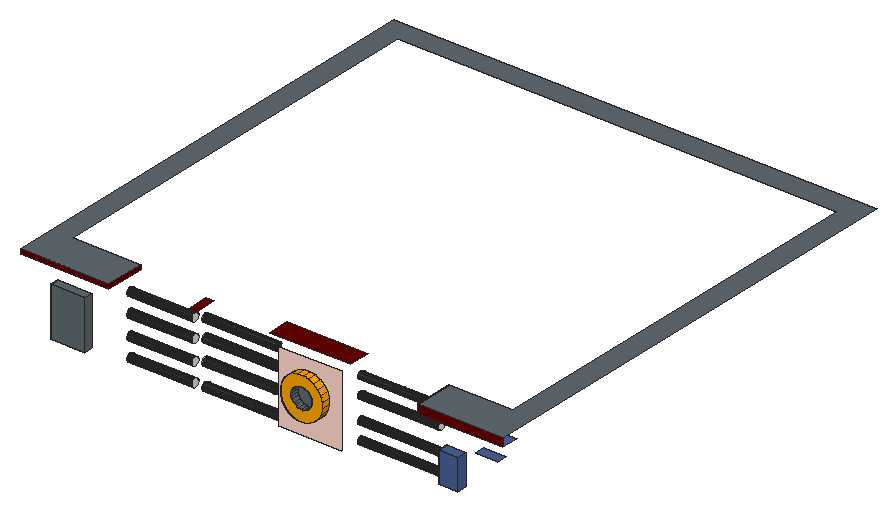
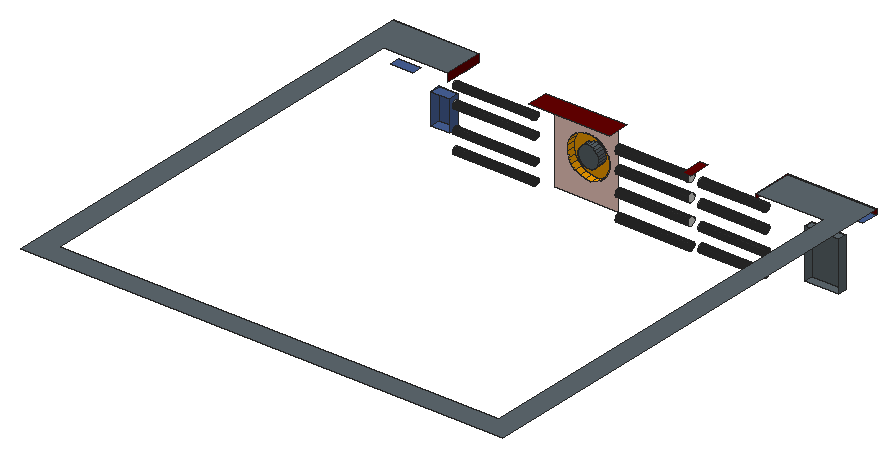
# SketchUp Ruby script. Lengths in inches.
U = 1.inch
M = Sketchup.active_model
def pt(a) = Geom::Point3d.new(a.map { |v| v * U })
def face(e, loops, mat)
  f = e.add_face(loops[0].map { |a| pt(a) })
  loops[1..].each { |l| e.add_face(l.map { |a| pt(a) }).erase! }
  f.material = f.back_material = mat if mat
  f
end
# faces: each face lists its corners as indices into pts; further lists are holes
def faces(e, pts, list, mat = nil) = list.each { |f| face(e, (f[0].is_a?(Array) ? f : [f]).map { |l| l.map { |i| pts[i] } }, mat) }
# xy, xz, yz: faces in a plane at the given z, y or x. An outline is a flat list of corners, or four numbers for a rectangle; further outlines are holes
def ring(l) = l.size == 4 ? [[l[0], l[1]], [l[2], l[1]], [l[2], l[3]], [l[0], l[3]]] : l.each_slice(2).to_a
def flat(e, list, mat, &to3) = list.each { |f| face(e, (f[0].is_a?(Array) ? f : [f]).map { |l| ring(l).map { |u, v| to3.(u, v) } }, mat) }
def xy(e, z, list, mat = nil) = flat(e, list, mat) { |x, y| [x, y, z] }
def xz(e, y, list, mat = nil) = flat(e, list, mat) { |x, z| [x, y, z] }
def yz(e, x, list, mat = nil) = flat(e, list, mat) { |y, z| [x, y, z] }
def lines(e, pts, list) = list.each { |a, b| e.add_line(pt(pts[a]), pt(pts[b])) }
# prism: a flat outline (further loops are holes) pulled along v
def prism(e, loops, v, mat = nil)
  f = face(e, loops, mat); d = Geom::Vector3d.new(v.map { |x| x * U })
  f.pushpull(f.normal.samedirection?(d) ? d.length : -d.length)
end
def box(e, o, s, mat = nil) = prism(e, [[o, [o[0] + s[0], o[1], o[2]], [o[0] + s[0], o[1] + s[1], o[2]], [o[0], o[1] + s[1], o[2]]]], [0, 0, s[2]], mat)
def at(x, y, z, deg = 0) = Geom::Transformation.translation(pt([x, y, z])) * Geom::Transformation.rotation(ORIGIN, Z_AXIS, deg.degrees)
def axes(o, x, y, z) = Geom::Transformation.new([*x, 0, *y, 0, *z, 0, *pt(o).to_a, 1])
def part(name) = M.definitions.add(name)
# library, detail: a bought-in or finely detailed component or shape, given as its bounding box
def library(name, o, s) = part(name).tap { |d| box(d.entities, o, s) }
def detail(e, o, s) = box(e.add_group.entities, o, s)
def put(e, d, t, mat = nil) = e.add_instance(d, t).tap { |i| i.material = mat if mat }
def group(e, t, mat = nil) = e.add_group.tap { |g| g.transformation = t; g.material = mat if mat }.entities
root = M.entities
M.materials.add("[0038_Orange]").color = [255, 165, 0]
M.materials.add("[Color A08]").color = [102, 0, 0]
M.materials.add("[Color B01]").color = [255, 216, 204]
M.materials.add("[Color M07]").color = [58, 58, 58]
M.materials.add("[Formica Blue]").color = [71, 97, 152]
M.materials.add("[Formica Speckled Grey]").color = [94, 105, 111]
xy(root,173.26,[[56.92,25.54,71.36,29.17]],"[Formica Speckled Grey]")
xy(root,176.39,[[221.42,24.73,229.42,29.17]],"[Formica Blue]")
xy(root,189.34,[[221.42,24.73,229.42,29.17]],"[Formica Blue]")
xy(root,193.75,[[236.96,24.73,246.46,29.17]],"[Formica Blue]")
xy(root,193.95,[[56.92,25.54,71.36,29.17]],"[Formica Speckled Grey]")
xy(root,200.34,[[198.48,33.52,198.76,33.56,199.01,33.66,199.23,33.83,199.4,34.05,199.51,34.31,199.55,34.58,199.51,34.86,199.4,35.12,199.23,35.34,199.01,35.5,198.76,35.61,198.48,35.65,198.21,35.61,197.95,35.5,197.73,35.34,197.5625,35.12,197.46,34.86,197.42,34.58,197.46,34.31,197.5625,34.05,197.73,33.83,197.95,33.66,198.21,33.56]])
xy(root,202.04,[[214.88,21.86,251.02,29.17]],"[Formica Blue]")
xy(root,202.625,[[112.25,29.17,115.75,38.27]],"[Color A08]")
xy(root,203.49,[[47,21.86,84.58,29.17]],"[Formica Blue]")
xy(root,205.625,[[146.64,29.17,180.76,38.27]],"[Color A08]")
xy(root,205.625,[[47,21.86,84.58,21.86,84.58,38.27,56.16,38.27,56.16,209.77,241.86,209.77,241.86,38.27,214.88,38.27,214.88,21.86,251.02,21.86,251.02,218.93,47,218.93]],"[Formica Speckled Grey]")
xz(root,21.86,[[214.88,202.04,251.02,205.625],[47,203.49,84.58,205.625]],"[Color A08]")
xz(root,24.73,[[221.42,176.39,229.42,189.34]],"[Formica Blue]")
xz(root,25.54,[[56.92,173.26,71.36,193.95]],"[Formica Speckled Grey]")
xz(root,25.67,[[[161.83,179.01,164.18,179.07,166.43,179.74,168.43,180.97,170.05,182.68,171.17,184.75,171.71,187.03,171.65,189.38,170.98,191.63,169.74,193.63,168.04,195.25,165.97,196.37,163.6875,196.91,161.34,196.85,159.09,196.17,157.08,194.94,155.47,193.24,154.35,191.17,153.81,188.89,153.87,186.54,154.54,184.29,155.77,182.28,157.48,180.67,159.55,179.55],[162.3,183.54,161.17,183.8,160.15,184.36,159.31,185.15,158.7,186.14,158.37,187.26,158.34,188.42,158.61,189.55,159.16,190.57,159.96,191.41,160.94,192.02,162.06,192.35,163.22,192.38,164.35,192.11,165.37,191.5625,166.21,190.76,166.82,189.77,167.15,188.66,167.18,187.5,166.91,186.37,166.36,185.35,165.5625,184.51,164.57,183.9,163.46,183.57]]],"[0038_Orange]")
xz(root,29.17,[[[150.55,171.54,176.84,201.71],[161.83,179.01,159.55,179.55,157.48,180.67,155.77,182.28,154.54,184.29,153.87,186.54,153.81,188.89,154.35,191.17,155.47,193.24,157.08,194.94,159.09,196.17,161.34,196.85,163.6875,196.91,165.97,196.37,168.04,195.25,169.74,193.63,170.98,191.63,171.65,189.38,171.71,187.03,171.17,184.75,170.05,182.68,168.43,180.97,166.43,179.74,164.18,179.07]]],"[Color B01]")
xz(root,29.17,[[162.3,183.54,163.46,183.57,164.57,183.9,165.5625,184.51,166.36,185.35,166.91,186.37,167.18,187.5,167.15,188.66,166.82,189.77,166.21,190.76,165.37,191.5625,164.35,192.11,163.22,192.38,162.06,192.35,160.94,192.02,159.96,191.41,159.16,190.57,158.61,189.55,158.34,188.42,158.37,187.26,158.7,186.14,159.31,185.15,160.15,184.36,161.17,183.8]],"[Formica Speckled Grey]")
yz(root,56.92,[[25.54,173.26,29.17,193.95]],"[Formica Speckled Grey]")
yz(root,71.36,[[25.54,173.26,29.17,193.95]],"[Formica Speckled Grey]")
yz(root,84.58,[[21.86,203.49,38.27,205.625]],"[Color A08]")
yz(root,112.25,[[32.81,171.26,33.23,171.3125,33.62,171.47,33.96,171.73,34.22,172.07,34.38,172.46,34.43,172.88,34.38,173.3,34.22,173.69,33.96,174.03,33.62,174.29,33.23,174.45,32.81,174.51,32.39,174.45,32,174.29,31.66,174.03,31.4,173.69,31.24,173.3,31.18,172.88,31.24,172.46,31.4,172.07,31.66,171.73,32,171.47,32.39,171.3125],[32.81,179.38,33.23,179.4375,33.62,179.6,33.96,179.86,34.22,180.19,34.38,180.59,34.43,181.01,34.38,181.43,34.22,181.82,33.96,182.16,33.62,182.41,33.23,182.58,32.81,182.63,32.39,182.58,32,182.41,31.66,182.16,31.4,181.82,31.24,181.43,31.18,181.01,31.24,180.59,31.4,180.19,31.66,179.86,32,179.6,32.39,179.4375],[32.81,188.01,33.23,188.0625,33.62,188.22,33.96,188.48,34.22,188.82,34.38,189.21,34.43,189.63,34.38,190.05,34.22,190.44,33.96,190.78,33.62,191.04,33.23,191.2,32.81,191.26,32.39,191.2,32,191.04,31.66,190.78,31.4,190.44,31.24,190.05,31.18,189.63,31.24,189.21,31.4,188.82,31.66,188.48,32,188.22,32.39,188.0625],[32.81,196.19,33.23,196.25,33.62,196.41,33.96,196.67,34.22,197.01,34.38,197.4,34.43,197.82,34.38,198.24,34.22,198.63,33.96,198.97,33.62,199.23,33.23,199.39,32.81,199.44,32.39,199.39,32,199.23,31.66,198.97,31.4,198.63,31.24,198.24,31.18,197.82,31.24,197.4,31.4,197.01,31.66,196.67,32,196.41,32.39,196.25]])
yz(root,115.75,[[33.57,180.44,33.15,180.5,32.76,180.66,32.42,180.92,32.17,181.26,32,181.65,31.95,182.07,32,182.49,32.17,182.88,32.42,183.22,32.76,183.48,33.15,183.64,33.57,183.69,33.99,183.64,34.39,183.48,34.72,183.22,34.98,182.88,35.14,182.49,35.2,182.07,35.14,181.65,34.98,181.26,34.72,180.92,34.39,180.66,33.99,180.5],[33.57,189.26,33.15,189.3125,32.76,189.47,32.42,189.73,32.17,190.07,32,190.46,31.95,190.88,32,191.3,32.17,191.69,32.42,192.03,32.76,192.29,33.15,192.45,33.57,192.51,33.99,192.45,34.39,192.29,34.72,192.03,34.98,191.69,35.14,191.3,35.2,190.88,35.14,190.46,34.98,190.07,34.72,189.73,34.39,189.47,33.99,189.3125],[33.57,196.94,33.15,197,32.76,197.16,32.42,197.42,32.17,197.76,32,198.15,31.95,198.57,32,198.99,32.17,199.38,32.42,199.72,32.76,199.98,33.15,200.14,33.57,200.19,33.99,200.14,34.39,199.98,34.72,199.72,34.98,199.38,35.14,198.99,35.2,198.57,35.14,198.15,34.98,197.76,34.72,197.42,34.39,197.16,33.99,197]])
yz(root,214.88,[[34.44,173.05,34.81,173.11,35.15,173.27,35.4375,173.51,35.66,173.82,35.79,174.17,35.82,174.54,35.76,174.91,35.6,175.25,35.36,175.54,35.05,175.76,34.7,175.89,34.33,175.92,33.96,175.86,33.62,175.7,33.33,175.46,33.11,175.16,32.98,174.8,32.95,174.43,33.01,174.06,33.17,173.72,33.41,173.43,33.71,173.21,34.07,173.08],[34.44,180.68,34.81,180.74,35.15,180.9,35.4375,181.14,35.66,181.44,35.79,181.8,35.82,182.17,35.76,182.54,35.6,182.88,35.36,183.17,35.05,183.38,34.7,183.51,34.33,183.55,33.96,183.48,33.62,183.33,33.33,183.09,33.11,182.78,32.98,182.43,32.95,182.06,33.01,181.69,33.17,181.34,33.41,181.06,33.71,180.84,34.07,180.71],[34.44,190.43,34.81,190.49,35.15,190.65,35.4375,190.89,35.66,191.19,35.79,191.55,35.82,191.92,35.76,192.29,35.6,192.63,35.36,192.92,35.05,193.13,34.7,193.26,34.33,193.3,33.96,193.23,33.62,193.08,33.33,192.84,33.11,192.53,32.98,192.18,32.95,191.81,33.01,191.44,33.17,191.09,33.41,190.81,33.71,190.59,34.07,190.46],[34.44,197.93,34.81,197.99,35.15,198.15,35.4375,198.39,35.66,198.69,35.79,199.05,35.82,199.42,35.76,199.79,35.6,200.13,35.36,200.42,35.05,200.63,34.7,200.76,34.33,200.8,33.96,200.73,33.62,200.58,33.33,200.34,33.11,200.03,32.98,199.68,32.95,199.31,33.01,198.94,33.17,198.59,33.41,198.31,33.71,198.09,34.07,197.96]])
yz(root,214.88,[[21.86,202.04,38.27,205.625]],"[Color A08]")
yz(root,221.42,[[24.73,176.39,29.17,189.34]],"[Formica Blue]")
yz(root,229.42,[[24.73,176.39,29.17,189.34]],"[Formica Blue]")
p = [[115.75,33.15,171],[115.75,33.57,170.94],[146.64,33.57,170.94],[146.64,33.15,171],[115.75,33.99,171],[146.64,33.99,171],
  [115.75,32.76,171.16],[146.64,32.76,171.16],[115.75,34.39,171.16],[146.64,34.39,171.16],[115.75,32.42,171.42],[146.64,32.42,171.42],
  [115.75,34.72,171.42],[146.64,34.72,171.42],[112.25,32.39,171.3125],[112.25,32,171.47],[84.58,32,171.47],[84.58,32.39,171.3125],
  [112.25,32.81,171.26],[84.58,32.81,171.26],[112.25,33.23,171.3125],[84.58,33.23,171.3125],[112.25,33.62,171.47],[84.58,33.62,171.47],
  [115.75,32.17,171.76],[146.64,32.17,171.76],[115.75,34.98,171.76],[146.64,34.98,171.76],[112.25,31.66,171.73],[84.58,31.66,171.73],
  [112.25,33.96,171.73],[84.58,33.96,171.73],[112.25,31.4,172.07],[84.58,31.4,172.07],[112.25,34.22,172.07],[84.58,34.22,172.07],
  [115.75,32,172.15],[146.64,32,172.15],[115.75,35.14,172.15],[146.64,35.14,172.15],[112.25,31.24,172.46],[84.58,31.24,172.46],
  [115.75,31.95,172.57],[146.64,31.95,172.57],[112.25,34.38,172.46],[84.58,34.38,172.46],[115.75,35.2,172.57],[146.64,35.2,172.57],
  [112.25,31.18,172.88],[84.58,31.18,172.88],[112.25,34.43,172.88],[84.58,34.43,172.88],[115.75,32,172.99],[146.64,32,172.99],
  [115.75,35.14,172.99],[146.64,35.14,172.99],[112.25,31.24,173.3],[84.58,31.24,173.3],[112.25,34.38,173.3],[84.58,34.38,173.3],
  [115.75,32.17,173.38],[146.64,32.17,173.38],[115.75,34.98,173.38],[146.64,34.98,173.38],[214.88,34.07,173.08],[214.88,33.71,173.21],
  [180.76,33.71,173.21],[180.76,34.07,173.08],[214.88,34.44,173.05],[180.76,34.44,173.05],[214.88,34.81,173.11],[180.76,34.81,173.11],
  [214.88,35.15,173.27],[180.76,35.15,173.27],[214.88,33.41,173.43],[180.76,33.41,173.43],[112.25,31.4,173.69],[84.58,31.4,173.69],
  [112.25,34.22,173.69],[84.58,34.22,173.69],[214.88,35.4375,173.51],[180.76,35.4375,173.51],[115.75,32.42,173.72],[146.64,32.42,173.72],
  [214.88,33.17,173.72],[180.76,33.17,173.72],[115.75,34.72,173.72],[146.64,34.72,173.72],[214.88,35.66,173.82],[180.76,35.66,173.82],
  [112.25,31.66,174.03],[84.58,31.66,174.03],[115.75,32.76,173.98],[146.64,32.76,173.98],[214.88,33.01,174.06],[180.76,33.01,174.06],
  [112.25,33.96,174.03],[84.58,33.96,174.03],[115.75,34.39,173.98],[146.64,34.39,173.98],[214.88,35.79,174.17],[180.76,35.79,174.17],
  [112.25,32,174.29],[84.58,32,174.29],[115.75,33.15,174.14],[146.64,33.15,174.14],[112.25,33.62,174.29],[84.58,33.62,174.29],
  [115.75,33.99,174.14],[146.64,33.99,174.14],[214.88,32.95,174.43],[180.76,32.95,174.43],[115.75,33.57,174.19],[146.64,33.57,174.19],
  [214.88,35.82,174.54],[180.76,35.82,174.54],[112.25,32.39,174.45],[84.58,32.39,174.45],[112.25,33.23,174.45],[84.58,33.23,174.45],
  [214.88,32.98,174.8],[180.76,32.98,174.8],[112.25,32.81,174.51],[84.58,32.81,174.51],[214.88,35.76,174.91],[180.76,35.76,174.91],
  [214.88,33.11,175.16],[180.76,33.11,175.16],[214.88,35.6,175.25],[180.76,35.6,175.25],[214.88,33.33,175.46],[180.76,33.33,175.46],
  [214.88,35.36,175.54],[180.76,35.36,175.54],[214.88,33.62,175.7],[180.76,33.62,175.7],[214.88,35.05,175.76],[180.76,35.05,175.76],
  [214.88,33.96,175.86],[180.76,33.96,175.86],[214.88,34.7,175.89],[180.76,34.7,175.89],[214.88,34.33,175.92],[180.76,34.33,175.92],
  [159.55,29.17,179.55],[161.83,29.17,179.01],[161.83,25.67,179.01],[159.55,25.67,179.55],[164.18,29.17,179.07],[164.18,25.67,179.07],
  [166.43,29.17,179.74],[166.43,25.67,179.74],[112.25,32.39,179.4375],[112.25,32,179.6],[84.58,32,179.6],[84.58,32.39,179.4375],
  [112.25,32.81,179.38],[84.58,32.81,179.38],[112.25,33.23,179.4375],[84.58,33.23,179.4375],[112.25,33.62,179.6],[84.58,33.62,179.6],
  [157.48,29.17,180.67],[157.48,25.67,180.67],[112.25,31.66,179.86],[84.58,31.66,179.86],[112.25,33.96,179.86],[84.58,33.96,179.86],
  [168.43,29.17,180.97],[168.43,25.67,180.97],[112.25,31.4,180.19],[84.58,31.4,180.19],[112.25,34.22,180.19],[84.58,34.22,180.19],
  [112.25,31.24,180.59],[84.58,31.24,180.59],[112.25,34.38,180.59],[84.58,34.38,180.59],[115.75,33.15,180.5],[115.75,33.57,180.44],
  [146.64,33.57,180.44],[146.64,33.15,180.5],[115.75,33.99,180.5],[146.64,33.99,180.5],[115.75,32.76,180.66],[146.64,32.76,180.66],
  [115.75,34.39,180.66],[146.64,34.39,180.66],[112.25,31.18,181.01],[84.58,31.18,181.01],[112.25,34.43,181.01],[84.58,34.43,181.01],
  [155.77,29.17,182.28],[155.77,25.67,182.28],[115.75,32.42,180.92],[146.64,32.42,180.92],[214.88,34.07,180.71],[214.88,33.71,180.84],
  [180.76,33.71,180.84],[180.76,34.07,180.71],[214.88,34.44,180.68],[180.76,34.44,180.68],[115.75,34.72,180.92],[146.64,34.72,180.92],
  [214.88,34.81,180.74],[180.76,34.81,180.74],[214.88,35.15,180.9],[180.76,35.15,180.9],[214.88,33.41,181.06],[180.76,33.41,181.06],
  [115.75,32.17,181.26],[146.64,32.17,181.26],[115.75,34.98,181.26],[146.64,34.98,181.26],[214.88,35.4375,181.14],[180.76,35.4375,181.14],
  [170.05,29.17,182.68],[170.05,25.67,182.68],[112.25,31.24,181.43],[84.58,31.24,181.43],[112.25,34.38,181.43],[84.58,34.38,181.43],
  [214.88,33.17,181.34],[180.76,33.17,181.34],[214.88,35.66,181.44],[180.76,35.66,181.44],[115.75,32,181.65],[146.64,32,181.65],
  [214.88,33.01,181.69],[180.76,33.01,181.69],[115.75,35.14,181.65],[146.64,35.14,181.65],[112.25,31.4,181.82],[84.58,31.4,181.82],
  [112.25,34.22,181.82],[84.58,34.22,181.82],[214.88,35.79,181.8],[180.76,35.79,181.8],[115.75,31.95,182.07],[146.64,31.95,182.07],
  [115.75,35.2,182.07],[146.64,35.2,182.07],[214.88,32.95,182.06],[180.76,32.95,182.06],[112.25,31.66,182.16],[84.58,31.66,182.16],
  [112.25,33.96,182.16],[84.58,33.96,182.16],[214.88,35.82,182.17],[180.76,35.82,182.17],[115.75,32,182.49],[146.64,32,182.49],
  [214.88,32.98,182.43],[180.76,32.98,182.43],[115.75,35.14,182.49],[146.64,35.14,182.49],[112.25,32,182.41],[84.58,32,182.41],
  [112.25,33.62,182.41],[84.58,33.62,182.41],[214.88,35.76,182.54],[180.76,35.76,182.54],[154.54,29.17,184.29],[154.54,25.67,184.29],
  [112.25,32.39,182.58],[84.58,32.39,182.58],[214.88,33.11,182.78],[180.76,33.11,182.78],[112.25,33.23,182.58],[84.58,33.23,182.58],
  [115.75,32.17,182.88],[146.64,32.17,182.88],[115.75,34.98,182.88],[146.64,34.98,182.88],[214.88,35.6,182.88],[180.76,35.6,182.88],
  [112.25,32.81,182.63],[84.58,32.81,182.63],[171.17,29.17,184.75],[171.17,25.67,184.75],[214.88,33.33,183.09],[180.76,33.33,183.09],
  [115.75,32.42,183.22],[146.64,32.42,183.22],[115.75,34.72,183.22],[146.64,34.72,183.22],[214.88,35.36,183.17],[180.76,35.36,183.17],
  [214.88,33.62,183.33],[180.76,33.62,183.33],[115.75,32.76,183.48],[146.64,32.76,183.48],[115.75,34.39,183.48],[146.64,34.39,183.48],
  [214.88,35.05,183.38],[180.76,35.05,183.38],[214.88,33.96,183.48],[180.76,33.96,183.48],[214.88,34.7,183.51],[180.76,34.7,183.51],
  [162.3,29.17,183.54],[161.17,29.17,183.8],[161.17,25.67,183.8],[162.3,25.67,183.54],[163.46,29.17,183.57],[163.46,25.67,183.57],
  [115.75,33.15,183.64],[146.64,33.15,183.64],[115.75,33.99,183.64],[146.64,33.99,183.64],[214.88,34.33,183.55],[180.76,34.33,183.55],
  [164.57,29.17,183.9],[164.57,25.67,183.9],[115.75,33.57,183.69],[146.64,33.57,183.69],[160.15,29.17,184.36],[160.15,25.67,184.36],
  [165.5625,29.17,184.51],[165.5625,25.67,184.51],[153.87,29.17,186.54],[153.87,25.67,186.54],[159.31,29.17,185.15],[159.31,25.67,185.15],
  [166.36,29.17,185.35],[166.36,25.67,185.35],[171.71,29.17,187.03],[171.71,25.67,187.03],[158.7,29.17,186.14],[158.7,25.67,186.14],
  [166.91,29.17,186.37],[166.91,25.67,186.37],[158.37,29.17,187.26],[158.37,25.67,187.26],[167.18,29.17,187.5],[167.18,25.67,187.5],
  [153.81,29.17,188.89],[153.81,25.67,188.89],[171.65,29.17,189.38],[171.65,25.67,189.38],[158.34,29.17,188.42],[158.34,25.67,188.42],
  [167.15,29.17,188.66],[167.15,25.67,188.66],[112.25,32.81,188.01],[112.25,32.39,188.0625],[84.58,32.39,188.0625],[84.58,32.81,188.01],
  [112.25,33.23,188.0625],[84.58,33.23,188.0625],[112.25,32,188.22],[84.58,32,188.22],[112.25,33.62,188.22],[84.58,33.62,188.22],
  [112.25,31.66,188.48],[84.58,31.66,188.48],[112.25,33.96,188.48],[84.58,33.96,188.48],[158.61,29.17,189.55],[158.61,25.67,189.55],
  [112.25,31.4,188.82],[84.58,31.4,188.82],[112.25,34.22,188.82],[84.58,34.22,188.82],[166.82,29.17,189.77],[166.82,25.67,189.77],
  [112.25,31.24,189.21],[84.58,31.24,189.21],[112.25,34.38,189.21],[84.58,34.38,189.21],[154.35,29.17,191.17],[154.35,25.67,191.17],
  [112.25,31.18,189.63],[84.58,31.18,189.63],[112.25,34.43,189.63],[84.58,34.43,189.63],[115.75,32.76,189.47],[115.75,33.15,189.3125],
  [146.64,33.15,189.3125],[146.64,32.76,189.47],[115.75,33.57,189.26],[146.64,33.57,189.26],[115.75,33.99,189.3125],[146.64,33.99,189.3125],
  [115.75,34.39,189.47],[146.64,34.39,189.47],[170.98,29.17,191.63],[170.98,25.67,191.63],[159.16,29.17,190.57],[159.16,25.67,190.57],
  [115.75,32.42,189.73],[146.64,32.42,189.73],[115.75,34.72,189.73],[146.64,34.72,189.73],[112.25,31.24,190.05],[84.58,31.24,190.05],
  [112.25,34.38,190.05],[84.58,34.38,190.05],[115.75,32.17,190.07],[146.64,32.17,190.07],[115.75,34.98,190.07],[146.64,34.98,190.07],
  [166.21,29.17,190.76],[166.21,25.67,190.76],[112.25,31.4,190.44],[84.58,31.4,190.44],[115.75,32,190.46],[146.64,32,190.46],
  [112.25,34.22,190.44],[84.58,34.22,190.44],[115.75,35.14,190.46],[146.64,35.14,190.46],[112.25,31.66,190.78],[84.58,31.66,190.78],
  [112.25,33.96,190.78],[84.58,33.96,190.78],[214.88,34.44,190.43],[214.88,34.07,190.46],[180.76,34.07,190.46],[180.76,34.44,190.43],
  [214.88,34.81,190.49],[180.76,34.81,190.49],[115.75,31.95,190.88],[146.64,31.95,190.88],[214.88,33.71,190.59],[180.76,33.71,190.59],
  [214.88,35.15,190.65],[180.76,35.15,190.65],[115.75,35.2,190.88],[146.64,35.2,190.88],[159.96,29.17,191.41],[159.96,25.67,191.41],
  [214.88,33.41,190.81],[180.76,33.41,190.81],[214.88,35.4375,190.89],[180.76,35.4375,190.89],[165.37,29.17,191.5625],[165.37,25.67,191.5625],
  [112.25,32,191.04],[84.58,32,191.04],[214.88,33.17,191.09],[180.76,33.17,191.09],[112.25,33.62,191.04],[84.58,33.62,191.04],
  [115.75,32,191.3],[146.64,32,191.3],[115.75,35.14,191.3],[146.64,35.14,191.3],[214.88,35.66,191.19],[180.76,35.66,191.19],
  [112.25,32.39,191.2],[84.58,32.39,191.2],[112.25,33.23,191.2],[84.58,33.23,191.2],[214.88,33.01,191.44],[180.76,33.01,191.44],
  [155.47,29.17,193.24],[155.47,25.67,193.24],[112.25,32.81,191.26],[84.58,32.81,191.26],[214.88,35.79,191.55],[180.76,35.79,191.55],
  [115.75,32.17,191.69],[146.64,32.17,191.69],[115.75,34.98,191.69],[146.64,34.98,191.69],[160.94,29.17,192.02],[160.94,25.67,192.02],
  [214.88,32.95,191.81],[180.76,32.95,191.81],[214.88,35.82,191.92],[180.76,35.82,191.92],[164.35,29.17,192.11],[164.35,25.67,192.11],
  [169.74,29.17,193.63],[169.74,25.67,193.63],[115.75,32.42,192.03],[146.64,32.42,192.03],[115.75,34.72,192.03],[146.64,34.72,192.03],
  [214.88,32.98,192.18],[180.76,32.98,192.18],[214.88,35.76,192.29],[180.76,35.76,192.29],[162.06,29.17,192.35],[162.06,25.67,192.35],
  [115.75,32.76,192.29],[146.64,32.76,192.29],[115.75,34.39,192.29],[146.64,34.39,192.29],[163.22,29.17,192.38],[163.22,25.67,192.38],
  [214.88,33.11,192.53],[180.76,33.11,192.53],[115.75,33.15,192.45],[146.64,33.15,192.45],[115.75,33.99,192.45],[146.64,33.99,192.45],
  [214.88,35.6,192.63],[180.76,35.6,192.63],[214.88,33.33,192.84],[180.76,33.33,192.84],[115.75,33.57,192.51],[146.64,33.57,192.51],
  [214.88,35.36,192.92],[180.76,35.36,192.92],[214.88,33.62,193.08],[180.76,33.62,193.08],[214.88,35.05,193.13],[180.76,35.05,193.13],
  [214.88,33.96,193.23],[180.76,33.96,193.23],[214.88,34.7,193.26],[180.76,34.7,193.26],[157.08,29.17,194.94],[157.08,25.67,194.94],
  [214.88,34.33,193.3],[180.76,34.33,193.3],[168.04,29.17,195.25],[168.04,25.67,195.25],[159.09,29.17,196.17],[159.09,25.67,196.17],
  [165.97,29.17,196.37],[165.97,25.67,196.37],[161.34,29.17,196.85],[161.34,25.67,196.85],[112.25,32.39,196.25],[112.25,32,196.41],
  [84.58,32,196.41],[84.58,32.39,196.25],[112.25,32.81,196.19],[84.58,32.81,196.19],[112.25,33.23,196.25],[84.58,33.23,196.25],
  [112.25,33.62,196.41],[84.58,33.62,196.41],[163.6875,29.17,196.91],[163.6875,25.67,196.91],[112.25,31.66,196.67],[84.58,31.66,196.67],
  [112.25,33.96,196.67],[84.58,33.96,196.67],[112.25,31.4,197.01],[84.58,31.4,197.01],[112.25,34.22,197.01],[84.58,34.22,197.01],
  [115.75,33.15,197],[115.75,33.57,196.94],[146.64,33.57,196.94],[146.64,33.15,197],[115.75,33.99,197],[146.64,33.99,197],
  [112.25,31.24,197.4],[84.58,31.24,197.4],[115.75,32.76,197.16],[146.64,32.76,197.16],[115.75,34.39,197.16],[146.64,34.39,197.16],
  [112.25,34.38,197.4],[84.58,34.38,197.4],[115.75,32.42,197.42],[146.64,32.42,197.42],[115.75,34.72,197.42],[146.64,34.72,197.42],
  [112.25,31.18,197.82],[84.58,31.18,197.82],[115.75,32.17,197.76],[146.64,32.17,197.76],[112.25,34.43,197.82],[84.58,34.43,197.82],
  [115.75,34.98,197.76],[146.64,34.98,197.76],[112.25,31.24,198.24],[84.58,31.24,198.24],[115.75,32,198.15],[146.64,32,198.15],
  [112.25,34.38,198.24],[84.58,34.38,198.24],[115.75,35.14,198.15],[146.64,35.14,198.15],[214.88,34.44,197.93],[214.88,34.07,197.96],
  [180.76,34.07,197.96],[180.76,34.44,197.93],[214.88,34.81,197.99],[180.76,34.81,197.99],[214.88,33.71,198.09],[180.76,33.71,198.09],
  [214.88,35.15,198.15],[180.76,35.15,198.15],[115.75,31.95,198.57],[146.64,31.95,198.57],[214.88,33.41,198.31],[180.76,33.41,198.31],
  [115.75,35.2,198.57],[146.64,35.2,198.57],[214.88,35.4375,198.39],[180.76,35.4375,198.39],[112.25,31.4,198.63],[84.58,31.4,198.63],
  [112.25,34.22,198.63],[84.58,34.22,198.63],[214.88,33.17,198.59],[180.76,33.17,198.59],[214.88,35.66,198.69],[180.76,35.66,198.69],
  [112.25,31.66,198.97],[84.58,31.66,198.97],[115.75,32,198.99],[146.64,32,198.99],[214.88,33.01,198.94],[180.76,33.01,198.94],
  [112.25,33.96,198.97],[84.58,33.96,198.97],[115.75,35.14,198.99],[146.64,35.14,198.99],[214.88,35.79,199.05],[180.76,35.79,199.05],
  [214.88,32.95,199.31],[180.76,32.95,199.31],[112.25,32,199.23],[84.58,32,199.23],[115.75,32.17,199.38],[146.64,32.17,199.38],
  [112.25,33.62,199.23],[84.58,33.62,199.23],[115.75,34.98,199.38],[146.64,34.98,199.38],[214.88,35.82,199.42],[180.76,35.82,199.42],
  [112.25,32.39,199.39],[84.58,32.39,199.39],[112.25,33.23,199.39],[84.58,33.23,199.39],[214.88,32.98,199.68],[180.76,32.98,199.68],
  [115.75,32.42,199.72],[146.64,32.42,199.72],[112.25,32.81,199.44],[84.58,32.81,199.44],[115.75,34.72,199.72],[146.64,34.72,199.72],
  [214.88,35.76,199.79],[180.76,35.76,199.79],[115.75,32.76,199.98],[146.64,32.76,199.98],[214.88,33.11,200.03],[180.76,33.11,200.03],
  [115.75,34.39,199.98],[146.64,34.39,199.98],[214.88,35.6,200.13],[180.76,35.6,200.13],[115.75,33.15,200.14],[146.64,33.15,200.14],
  [214.88,33.33,200.34],[180.76,33.33,200.34],[115.75,33.99,200.14],[146.64,33.99,200.14],[115.75,33.57,200.19],[146.64,33.57,200.19],
  [214.88,35.36,200.42],[180.76,35.36,200.42],[214.88,33.62,200.58],[180.76,33.62,200.58],[214.88,35.05,200.63],[180.76,35.05,200.63],
  [214.88,33.96,200.73],[180.76,33.96,200.73],[214.88,34.7,200.76],[180.76,34.7,200.76],[214.88,34.33,200.8],[180.76,34.33,200.8]]
faces(root,p,[[0,1,2,3],[1,4,5,2],[6,0,3,7],[4,8,9,5],[10,6,7,11],[8,12,13,9],[14,15,16,17],[18,14,17,19],
  [20,18,19,21],[22,20,21,23],[24,10,11,25],[12,26,27,13],[15,28,29,16],[30,22,23,31],[28,32,33,29],[34,30,31,35],
  [36,24,25,37],[26,38,39,27],[32,40,41,33],[42,36,37,43],[44,34,35,45],[38,46,47,39],[40,48,49,41],[50,44,45,51],
  [52,42,43,53],[46,54,55,47],[48,56,57,49],[58,50,51,59],[60,52,53,61],[54,62,63,55],[64,65,66,67],[68,64,67,69],
  [70,68,69,71],[72,70,71,73],[65,74,75,66],[56,76,77,57],[78,58,59,79],[80,72,73,81],[82,60,61,83],[74,84,85,75],
  [62,86,87,63],[88,80,81,89],[76,90,91,77],[92,82,83,93],[84,94,95,85],[96,78,79,97],[86,98,99,87],[100,88,89,101],
  [90,102,103,91],[104,92,93,105],[106,96,97,107],[98,108,109,99],[94,110,111,95],[112,104,105,113],[108,112,113,109],[114,100,101,115],
  [102,116,117,103],[118,106,107,119],[110,120,121,111],[116,122,123,117],[122,118,119,123],[124,114,115,125],[120,126,127,121],[128,124,125,129],
  [126,130,131,127],[132,128,129,133],[130,134,135,131],[136,132,133,137],[134,138,139,135],[140,136,137,141],[138,142,143,139],[142,140,141,143],
  [152,153,154,155],[156,152,155,157],[158,156,157,159],[160,158,159,161],[153,164,165,154],[166,160,161,167],[164,170,171,165],[172,166,167,173],
  [170,174,175,171],[176,172,173,177],[178,179,180,181],[179,182,183,180],[184,178,181,185],[182,186,187,183],[174,188,189,175],[190,176,177,191],
  [194,184,185,195],[196,197,198,199],[200,196,199,201],[186,202,203,187],[204,200,201,205],[206,204,205,207],[197,208,209,198],[210,194,195,211],
  [202,212,213,203],[214,206,207,215],[188,218,219,189],[220,190,191,221],[208,222,223,209],[224,214,215,225],[226,210,211,227],[222,228,229,223],
  [212,230,231,213],[218,232,233,219],[234,220,221,235],[236,224,225,237],[238,226,227,239],[230,240,241,231],[228,242,243,229],[232,244,245,233],
  [246,234,235,247],[248,236,237,249],[250,238,239,251],[242,252,253,243],[240,254,255,241],[244,256,257,245],[258,246,247,259],[260,248,249,261],
  [256,264,265,257],[252,266,267,253],[268,258,259,269],[270,250,251,271],[254,272,273,255],[274,260,261,275],[264,276,277,265],[276,268,269,277],
  [266,280,281,267],[282,270,271,283],[272,284,285,273],[286,274,275,287],[280,288,289,281],[290,282,283,291],[284,292,293,285],[294,286,287,295],
  [288,296,297,289],[298,294,295,299],[306,290,291,307],[292,308,309,293],[296,310,311,297],[310,298,299,311],[314,306,307,315],[308,314,315,309],
  [344,345,346,347],[348,344,347,349],[345,350,351,346],[352,348,349,353],[350,354,355,351],[356,352,353,357],[354,360,361,355],[362,356,357,363],
  [360,366,367,361],[368,362,363,369],[366,372,373,367],[374,368,369,375],[376,377,378,379],[377,380,381,378],[380,382,383,381],[382,384,385,383],
  [390,376,379,391],[384,392,393,385],[372,394,395,373],[396,374,375,397],[398,390,391,399],[392,400,401,393],[394,404,405,395],[406,398,399,407],
  [408,396,397,409],[400,410,411,401],[404,412,413,405],[414,408,409,415],[416,417,418,419],[420,416,419,421],[422,406,407,423],[417,424,425,418],
  [426,420,421,427],[410,428,429,411],[424,432,433,425],[434,426,427,435],[412,438,439,413],[432,440,441,433],[442,414,415,443],[444,422,423,445],
  [428,446,447,429],[448,434,435,449],[438,450,451,439],[452,442,443,453],[440,454,455,441],[450,458,459,451],[458,452,453,459],[460,448,449,461],
  [462,444,445,463],[446,464,465,447],[454,468,469,455],[470,460,461,471],[476,462,463,477],[464,478,479,465],[468,480,481,469],[482,470,471,483],
  [486,476,477,487],[478,488,489,479],[480,492,493,481],[494,486,487,495],[488,496,497,489],[498,482,483,499],[492,500,501,493],[502,494,495,503],
  [496,502,503,497],[504,498,499,505],[500,506,507,501],[508,504,505,509],[506,510,511,507],[512,508,509,513],[510,516,517,511],[516,512,513,517],
  [526,527,528,529],[530,526,529,531],[532,530,531,533],[534,532,533,535],[527,538,539,528],[540,534,535,541],[538,542,543,539],[544,540,541,545],
  [546,547,548,549],[547,550,551,548],[542,552,553,543],[554,546,549,555],[550,556,557,551],[558,544,545,559],[560,554,555,561],[556,562,563,557],
  [552,564,565,553],[566,560,561,567],[568,558,559,569],[562,570,571,563],[564,572,573,565],[574,566,567,575],[576,568,569,577],[570,578,579,571],
  [580,581,582,583],[584,580,583,585],[581,586,587,582],[588,584,585,589],[590,574,575,591],[586,592,593,587],[578,594,595,579],[596,588,589,597],
  [572,598,599,573],[600,576,577,601],[592,602,603,593],[604,596,597,605],[598,606,607,599],[608,590,591,609],[602,610,611,603],[612,600,601,613],
  [594,614,615,595],[616,604,605,617],[610,618,619,611],[606,620,621,607],[622,608,609,623],[624,612,613,625],[614,626,627,615],[628,616,617,629],
  [620,630,631,621],[632,624,625,633],[618,634,635,619],[636,622,623,637],[630,638,639,631],[638,632,633,639],[626,640,641,627],[642,628,629,643],
  [644,636,637,645],[634,646,647,635],[640,648,649,641],[650,642,643,651],[652,644,645,653],[646,654,655,647],[648,656,657,649],[658,652,653,659],
  [656,658,659,657],[660,650,651,661],[654,662,663,655],[664,660,661,665],[662,666,667,663],[668,664,665,669],[666,670,671,667],[670,668,669,671]],"[Color M07]")
faces(root,p,[[144,145,146,147],[145,148,149,146],[148,150,151,149],[162,144,147,163],[150,168,169,151],[192,162,163,193],[168,216,217,169],[262,192,193,263],
  [216,278,279,217],[320,262,263,321],[278,326,327,279],[336,320,321,337],[326,338,339,327],[370,336,337,371],[338,386,387,339],[456,370,371,457],
  [386,474,475,387],[514,456,457,515],[474,518,519,475],[520,514,515,521],[518,522,523,519],[524,520,521,525],[522,536,537,523],[536,524,525,537]],"[0038_Orange]")
faces(root,p,[[300,301,302,303],[304,300,303,305],[312,304,305,313],[301,316,317,302],[318,312,313,319],[316,322,323,317],[324,318,319,325],[322,328,329,323],
  [330,324,325,331],[328,332,333,329],[334,330,331,335],[332,340,341,333],[342,334,335,343],[340,358,359,341],[364,342,343,365],[358,388,389,359],
  [402,364,365,403],[388,430,431,389],[436,402,403,437],[430,466,467,431],[472,436,437,473],[466,484,485,467],[490,472,473,491],[484,490,491,485]],"[Formica Speckled Grey]")
